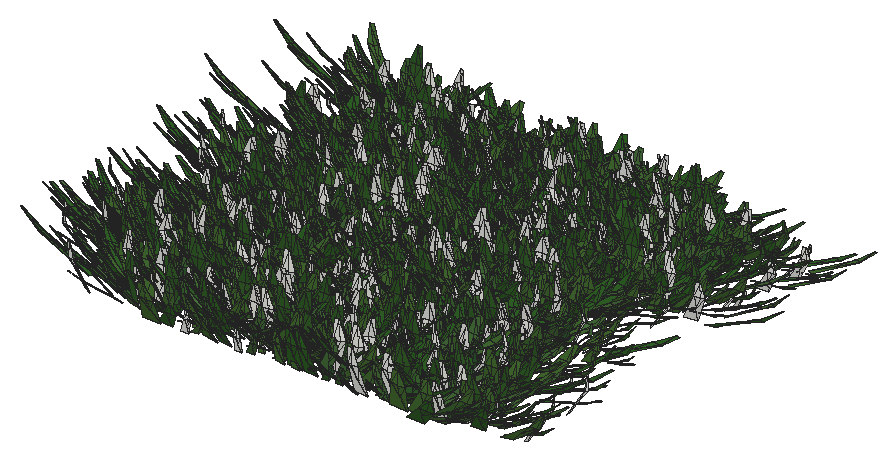
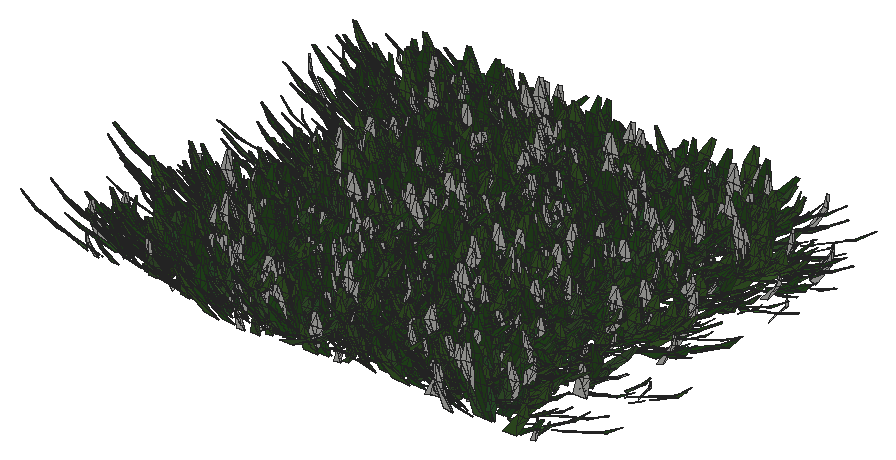
# SketchUp Ruby script. Lengths in inches.
U = 1.inch
M = Sketchup.active_model
def pt(a) = Geom::Point3d.new(a.map { |v| v * U })
def face(e, loops, mat)
  f = e.add_face(loops[0].map { |a| pt(a) })
  loops[1..].each { |l| e.add_face(l.map { |a| pt(a) }).erase! }
  f.material = f.back_material = mat if mat
  f
end
# faces: each face lists its corners as indices into pts; further lists are holes
def faces(e, pts, list, mat = nil) = list.each { |f| face(e, (f[0].is_a?(Array) ? f : [f]).map { |l| l.map { |i| pts[i] } }, mat) }
# xy, xz, yz: faces in a plane at the given z, y or x. An outline is a flat list of corners, or four numbers for a rectangle; further outlines are holes
def ring(l) = l.size == 4 ? [[l[0], l[1]], [l[2], l[1]], [l[2], l[3]], [l[0], l[3]]] : l.each_slice(2).to_a
def flat(e, list, mat, &to3) = list.each { |f| face(e, (f[0].is_a?(Array) ? f : [f]).map { |l| ring(l).map { |u, v| to3.(u, v) } }, mat) }
def xy(e, z, list, mat = nil) = flat(e, list, mat) { |x, y| [x, y, z] }
def xz(e, y, list, mat = nil) = flat(e, list, mat) { |x, z| [x, y, z] }
def yz(e, x, list, mat = nil) = flat(e, list, mat) { |y, z| [x, y, z] }
def lines(e, pts, list) = list.each { |a, b| e.add_line(pt(pts[a]), pt(pts[b])) }
# prism: a flat outline (further loops are holes) pulled along v
def prism(e, loops, v, mat = nil)
  f = face(e, loops, mat); d = Geom::Vector3d.new(v.map { |x| x * U })
  f.pushpull(f.normal.samedirection?(d) ? d.length : -d.length)
end
def box(e, o, s, mat = nil) = prism(e, [[o, [o[0] + s[0], o[1], o[2]], [o[0] + s[0], o[1] + s[1], o[2]], [o[0], o[1] + s[1], o[2]]]], [0, 0, s[2]], mat)
def at(x, y, z, deg = 0) = Geom::Transformation.translation(pt([x, y, z])) * Geom::Transformation.rotation(ORIGIN, Z_AXIS, deg.degrees)
def axes(o, x, y, z) = Geom::Transformation.new([*x, 0, *y, 0, *z, 0, *pt(o).to_a, 1])
def part(name) = M.definitions.add(name)
# library, detail: a bought-in or finely detailed component or shape, given as its bounding box
def library(name, o, s) = part(name).tap { |d| box(d.entities, o, s) }
def detail(e, o, s) = box(e.add_group.entities, o, s)
def put(e, d, t, mat = nil) = e.add_instance(d, t).tap { |i| i.material = mat if mat }
def group(e, t, mat = nil) = e.add_group.tap { |g| g.transformation = t; g.material = mat if mat }.entities
root = M.entities
M.materials.add("Material10").color = [48, 100, 38]
M.materials.add("Material3").color = [68, 110, 58]
M.materials.add("Material4").color = [48, 90, 38]
M.materials.add("Material5").color = [68, 110, 48]
M.materials.add("Material6").color = [48, 90, 48]
M.materials.add("Material7").color = [58, 110, 58]
M.materials.add("Material8").color = [58, 90, 38]
M.materials.add("Material9").color = [68, 100, 58]
c1 = part("grass00")
p = [[-0.6875,0.15,0],[-0.56,0.08,5.52],[-0.04,0.03,2.76],[0.48,-0.02,0],[0.35,-0.02,5.52],[-0.1,-0.14,5.52],
  [-0.12,0.65,8.37],[-0.42,0.65,8.37]]
faces(c1.entities,p,[[0,1,2,3],[3,2,4],[1,5,2],[5,4,2],[1,6,5],[4,5,6],[7,6,1]])
c2 = part("Group16\#1")
put(c2.entities,c1,axes([1.44,-0.61,-0.01],[0.05352,0.12609,0],[-0.10704,0.04543,0.07239],[0.06664,-0.02828,0.11628]),"Material6")
put(c2.entities,c1,axes([0.76,-0.15,-0.01],[0.04676,0.24062,0],[-0.23162,0.04501,0.06642],[0.0652,-0.01267,0.23595]),"Material3")
put(c2.entities,c1,axes([0.79,0.01,-0.01],[-0.00606,0.34651,0],[-0.34381,-0.00602,0.0432],[0.04319,0.00076,0.34386]))
put(c2.entities,c1,axes([1,0.23,-0.01],[-0.07192,0.31144,0],[-0.28722,-0.06632,0.1236],[0.12043,0.02781,0.29478]),"Material5")
put(c2.entities,c1,axes([1.66,0.77,-0.01],[-0.13828,0.29651,0],[-0.21551,-0.1005,0.22471],[0.20365,0.09498,0.23779]),"Material10")
put(c2.entities,c1,axes([0.6875,0.52,-0.01],[-0.18126,0.24051,0],[-0.22746,-0.17142,0.09788],[0.07817,0.05891,0.28481]),"Material5")
put(c2.entities,c1,axes([0.68,0.78,-0.01],[-0.215,0.18688,0],[-0.12385,-0.14248,0.21334],[0.13995,0.16101,0.18878]),"Material3")
put(c2.entities,c1,axes([0.56,1,-0.01],[-0.13756,0.07624,0],[-0.06159,-0.11112,0.0927],[0.04494,0.08108,0.12705]),"Material5")
put(c2.entities,c1,axes([0.2,0.64,-0.01],[-0.23729,0.07254,0],[-0.05711,-0.18681,0.153],[0.04473,0.14632,0.19535]),"Material10")
put(c2.entities,c1,axes([0.0625,0.72,-0.01],[-0.28874,0.02525,0],[-0.02179,-0.24916,0.14647],[0.01276,0.14591,0.25012]),"Material3")
put(c2.entities,c1,axes([-0.08,0.62,-0.01],[-0.34089,-0.04187,0],[0.03255,-0.26504,0.216],[-0.02633,0.21439,0.26703]),"Material10")
put(c2.entities,c1,axes([-0.34,0.98,-0.01],[-0.14314,-0.0493,0],[0.04397,-0.12769,0.06843],[-0.02228,0.0647,0.13505]),"Material10")
put(c2.entities,c1,axes([-0.87,1.45,-0.01],[-0.23488,-0.14114,0],[0.13761,-0.22901,0.06087],[-0.03135,0.05217,0.26717]))
put(c2.entities,c1,axes([-0.72,0.77,-0.01],[-0.14208,-0.13251,0],[0.07209,-0.0773,0.16301],[-0.11118,0.11922,0.1057]),"Material10")
put(c2.entities,c1,axes([-0.62,0.43,-0.01],[-0.14845,-0.21203,0],[0.18654,-0.13061,0.12304],[-0.10079,0.07057,0.22772]),"Material3")
put(c2.entities,c1,axes([-0.68,0.29,-0.01],[-0.13639,-0.32136,0],[0.31723,-0.13464,0.05579],[-0.05136,0.0218,0.34462]),"Material4")
put(c2.entities,c1,axes([-0.64,0.125,-0.01],[-0.0458,-0.23569,0],[0.22124,-0.043,0.08276],[-0.08124,0.01579,0.22538]),"Material7")
put(c2.entities,c1,axes([-1.6,-0.03,-0.01],[0.00576,-0.32897,0],[0.27526,0.00482,0.18018],[-0.18015,-0.00315,0.2753]),"Material5")
put(c2.entities,c1,axes([-1.36,-0.31,-0.01],[0.05718,-0.24765,0],[0.18172,0.04196,0.17267],[-0.16825,-0.03885,0.1865]),"Material10")
put(c2.entities,c1,axes([-1.54,-0.72,-0.01],[0.06537,-0.14017,0],[0.13555,0.06321,0.03939],[-0.0357,-0.01665,0.14956]))
put(c2.entities,c1,axes([-1.19,-0.9,-0.01],[0.09597,-0.12735,0],[0.11214,0.08451,0.07557],[-0.06035,-0.04548,0.14042]),"Material9")
put(c2.entities,c1,axes([-0.47,-0.54,-0.01],[0.11588,-0.10072,0],[0.0618,0.0711,0.12124],[-0.07953,-0.0915,0.0942]))
put(c2.entities,c1,axes([-0.47,-0.84,-0.01],[0.11927,-0.0661,0],[0.06603,0.11913,0.00646],[-0.00313,-0.00565,0.13621]),"Material5")
put(c2.entities,c1,axes([-0.38,-1.24,-0.01],[0.28037,-0.08571,0],[0.0618,0.20215,0.20315],[-0.05939,-0.19428,0.21139]),"Material9")
put(c2.entities,c1,axes([-0.06,-0.66,-0.01],[0.22719,-0.01987,0],[0.01247,0.14255,0.17758],[-0.01547,-0.17691,0.1431]),"Material8")
put(c2.entities,c1,axes([0.11,-0.89,-0.01],[0.14882,0.01828,0],[-0.01058,0.08611,0.12229],[0.01491,-0.12138,0.08676]),"Material6")
put(c2.entities,c1,axes([0.25,-0.72,-0.01],[0.20481,0.07053,0],[-0.06206,0.18022,0.10291],[0.03351,-0.0973,0.1906]),"Material6")
put(c2.entities,c1,axes([0.85,-1.42,-0.01],[0.16481,0.09904,0],[-0.09472,0.15762,0.05616],[0.02893,-0.04814,0.18389]),"Material5")
put(c2.entities,c1,axes([1.01,-1.09,-0.01],[0.21858,0.20385,0],[-0.17495,0.1876,0.15339],[0.10462,-0.11218,0.25652]),"Material10")
put(c2.entities,c1,axes([1.01,-0.71,-0.01],[0.08733,0.12473,0],[-0.06445,0.04512,0.13037],[0.1068,-0.07477,0.07867]),"Material6")
c3 = part("Group15\#1")
put(c3.entities,c2,at(0,0,0))
c4 = part("3darcstudiotree_grass00\#1")
put(c4.entities,c3,at(0,0,0))
put(root,c4,axes([955.85,939.92,0],[-0.75214,1.19237,0],[-4.74693,-0.18715,-0.03641],[-0.174,-0.00686,1.45326]))
put(root,c4,axes([955.95,963.41,0],[4.69551,-0.08423,0],[0.3605,1.25607,-0.01186],[0.0041,0.0143,1.52253]))
put(root,c4,axes([956.82,972.28,0],[2.38234,-0.95226,0],[3.20328,0.50086,-0.0272],[0.17769,0.02778,1.81972]))
put(root,c4,axes([956.31,940.49,0],[-1.46228,1.23307,0],[-3.47122,-0.25728,-0.00114],[-0.00907,-0.00067,1.86907]))
put(root,c4,axes([955.81,946.5,0],[1.47006,1.1325,0],[-4.40979,0.35776,-0.01715],[-0.07948,0.00645,1.41194]))
put(root,c4,axes([957,953.02,0],[-2.07415,0.83506,0],[-3.95028,-0.61324,-0.02009],[-0.09896,-0.01536,1.68525]))
put(root,c4,axes([957.88,954.94,0],[-1.18382,1.15457,0],[-4.70826,-0.30172,-0.05431],[-0.29177,-0.0187,1.6847]))
put(root,c4,axes([958.3,969.83,0],[-3.28461,0.98923,0],[-3.37325,-0.70003,-0.00469],[-0.02101,-0.00436,1.59556]))
put(root,c4,axes([957.74,956.29,0],[2.88148,0.64126,0],[-3.12484,0.87758,-0.03405],[-0.12784,0.0359,1.65877]))
put(root,c4,axes([958.03,942.36,0],[3.07935,0.60729,0],[-3.11371,0.98678,-0.06164],[-0.16424,0.05205,1.3518]))
put(root,c4,axes([958.4,937.74,0],[0.52678,1.06322,0],[-4.94177,0.15303,-0.03401],[-0.15238,0.00472,1.40523]))
put(root,c4,axes([960.7,959.67,0],[1.39418,-0.83958,0],[3.77377,0.39166,-0.03248],[0.18939,0.01966,1.61223]))
put(root,c4,axes([961.12,949.46,0],[-4.00371,0.05544,0],[-0.23957,-1.08136,-0.04105],[-0.01536,-0.06935,1.83253]))
put(root,c4,axes([960.22,961.01,0],[-0.74123,1.26839,0],[-3.97906,-0.14533,-0.03578],[-0.18887,-0.0069,1.34076]))
put(root,c4,axes([961.14,934.34,0],[-3.45273,0.48202,0],[-2.12645,-0.95198,-0.05669],[-0.18901,-0.08462,1.86391]))
put(root,c4,axes([961.79,942.36,0],[-2.58874,-0.9071,0],[3.15855,-0.56338,-0.04134],[0.26965,-0.0481,1.943]))
put(root,c4,axes([961,938.43,0],[-3.19228,0.66883,0],[-3.28024,-0.97852,-0.01682],[-0.06095,-0.01818,1.80026]))
put(root,c4,axes([961.375,964.91,0],[-3.68677,0.78294,0],[-2.37097,-0.69779,-0.00331],[-0.01382,-0.00407,1.47415]))
put(root,c4,axes([961.87,941.45,0],[2.79001,-0.91126,0],[3.28074,0.62779,-0.00025],[0.00114,0.00022,1.45509]))
put(root,c4,axes([961.69,951.44,0],[3.11012,-0.98955,0],[3.48139,0.68387,-0.04001],[0.20872,0.041,1.83572]))
put(root,c4,axes([960.94,947.1,0],[4.49844,0.3136,0],[-1.0523,0.94343,-0.03867],[-0.07449,0.06678,1.75619]))
put(root,c4,axes([961.3,966.6875,0],[0.32984,1.08986,0],[-4.10586,0.07766,-0.04286],[-0.23653,0.00447,1.42447]))
put(root,c4,axes([963.09,945.71,0],[-3.31262,-0.80999,0],[3.0672,-0.784,-0.0483],[0.19534,-0.04993,1.58573]))
put(root,c4,axes([962.21,968.11,0],[3.83987,-0.74679,0],[3.08152,0.9903,-0.05588],[0.18273,0.05872,1.67045]))
put(root,c4,axes([961.67,933.4,0],[-0.43739,1.1748,0],[-4.7805,-0.11124,-0.02425],[-0.1421,-0.00331,1.76617]))
put(root,c4,axes([963.72,970.83,0],[-1.00327,-1.08198,0],[4.89707,-0.2838,-0.01344],[0.05958,-0.00345,1.42931]))
put(root,c4,axes([962.97,957.125,0],[-4.17134,0.59694,0],[-1.91655,-0.83704,-0.03218],[-0.1099,-0.048,1.65786]))
put(root,c4,axes([963.5625,936.91,0],[1.82974,-1.11236,0],[4.14269,0.4259,-0.00107],[0.00497,0.00051,1.41133]))
put(root,c4,axes([962.8,969.7,0],[-2.1717,0.94775,0],[-3.61053,-0.51708,-0.00674],[-0.03293,-0.00472,1.46389]))
put(root,c4,axes([963.11,943.8,0],[-1.78952,0.96069,0],[-3.60864,-0.42012,-0.01596],[-0.10849,-0.01263,1.86544]))
put(root,c4,axes([963.37,948.01,0],[-2.06309,0.87153,0],[-4.13288,-0.61146,-0.04665],[-0.19777,-0.02926,1.47851]))
put(root,c4,axes([964.55,964.07,0],[-3.51429,-0.45659,0],[1.66461,-0.80077,-0.02241],[0.07721,-0.03714,1.68548]))
put(root,c4,axes([963.58,956.58,0],[2.73197,0.7121,0],[-2.97454,0.71324,-0.02632],[-0.14399,0.03453,1.95302]))
put(root,c4,axes([963.97,961.88,0],[4.48019,-0.41485,0],[1.31658,0.88866,-0.03178],[0.08406,0.05674,1.80429]))
put(root,c4,axes([963.76,939.38,0],[2.54094,0.64898,0],[-3.14239,0.76896,-0.01876],[-0.08636,0.02113,1.77063]))
put(root,c4,axes([964.56,952.54,0],[0.1997,1.06432,0],[-4.51312,0.05293,-0.04808],[-0.29009,0.0034,1.70557]))
put(root,c4,axes([963.97,955,0],[1.85724,1.07697,0],[-4.66485,0.50278,-0.01792],[-0.06948,0.00749,1.34035]))
put(root,c4,axes([966.91,963.85,0],[-1.0135,-1.00462,0],[4.08606,-0.25764,-0.02503],[0.13624,-0.00859,1.47852]))
put(root,c4,axes([966.41,943.59,0],[-4.005,0.7272,0],[-2.3018,-0.79231,-0.02785],[-0.12344,-0.04249,1.84622]))
put(root,c4,axes([966.39,951.57,0],[2.95335,-0.82152,0],[2.70823,0.6085,-0.01288],[0.06524,0.01466,1.54961]))
put(root,c4,axes([967.34,946.85,0],[-4.20956,-0.26717,0],[1.18231,-1.16431,-0.00944],[0.01496,-0.01473,1.93444]))
put(root,c4,axes([967.17,942.34,0],[-1.13661,-1.06386,0],[4.15271,-0.27729,-0.04991],[0.23787,-0.01588,1.32514]))
put(root,c4,axes([967.32,941.08,0],[2.16693,-1.10955,0],[3.94511,0.48154,-0.03421],[0.21213,0.02589,1.89316]))
put(root,c4,axes([966.46,953.29,0],[1.18,1.03822,0],[-4.57121,0.32472,-0.01918],[-0.11705,0.00831,1.88463]))
put(root,c4,axes([968.1,962.44,0],[-3.50507,0.61445,0],[-2.29769,-0.81919,-0.04222],[-0.17037,-0.06074,1.75818]))
put(root,c4,axes([969.18,959.26,0],[-3.58509,-0.60969,0],[2.592,-0.9526,-0.01911],[0.04957,-0.01822,1.32815]))
put(root,c4,axes([968.8125,939.43,0],[-0.06451,-0.92143,0],[4.54272,-0.01988,-0.04239],[0.21245,-0.00093,1.42343]))
put(root,c4,axes([968.87,965,0],[-4.03446,-0.01635,0],[0.06659,-1.02672,-0.00434],[0.00038,-0.00582,1.37632]))
put(root,c4,axes([967.4375,971.16,0],[3.92463,0.27646,0],[-1.34669,1.19487,-0.04858],[-0.06681,0.05928,1.57379]))
put(root,c4,axes([969.7,950.29,0],[-0.14207,-1.06089,0],[4.63971,-0.03883,-0.02714],[0.13515,-0.00113,1.44559]))
put(root,c4,axes([969.22,956.53,0],[-4.11295,0.48392,0],[-1.88318,-1.00036,-0.0027],[-0.00657,-0.00349,1.57765]))
put(root,c4,axes([969.27,969.92,0],[-3.01374,0.50325,0],[-2.28022,-0.85345,-0.04884],[-0.14675,-0.05493,1.38796]))
put(root,c4,axes([969.28,935.29,0],[2.85144,-0.93309,0],[3.29337,0.62902,-0.00592],[0.03247,0.0062,1.78738]))
put(root,c4,axes([970.22,936.01,0],[-2.85912,-0.7944,0],[3.18267,-0.71592,-0.02928],[0.11058,-0.02487,1.35967]))
put(root,c4,axes([970.48,967.84,0],[-4.01975,-0.67401,0],[2.06418,-0.76941,-0.03319],[0.1306,-0.04868,1.63594]))
put(root,c4,axes([969.0625,960.27,0],[-0.9226,1.08456,0],[-4.51637,-0.24012,-0.02719],[-0.16539,-0.00879,1.79436]))
put(root,c4,axes([969.36,954.06,0],[-0.15668,0.99341,0],[-4.74141,-0.04674,-0.01193],[-0.07952,-0.00078,1.97773]))
put(root,c4,axes([970.32,957.8,0],[-0.75974,1.09038,0],[-3.60462,-0.15698,-0.03897],[-0.29833,-0.01299,1.77692]))
put(root,c4,axes([970.2,945.88,0],[-0.10594,0.90385,0],[-3.73304,-0.02735,-0.04664],[-0.28296,-0.00207,1.41669]))
put(root,c4,axes([969.74,933.68,0],[1.08855,0.96574,0],[-4.18203,0.29461,-0.02067],[-0.12416,0.00875,1.69495]))
put(root,c4,axes([970.14,949.04,0],[3.05692,0.87665,0],[-2.75486,0.6004,-0.0286],[-0.17096,0.03726,1.81122]))
put(root,c4,axes([970.41,938.2,0],[-0.61059,1.1553,0],[-4.99702,-0.16506,-0.03274],[-0.14868,-0.00491,1.44297]))
put(root,c4,axes([970.23,966.68,0],[4.02977,0.69816,0],[-2.76519,0.99754,-0.01195],[-0.03084,0.01113,1.37528]))
put(root,c4,axes([972.49,959.14,0],[-4.6224,0.20326,0],[-0.67084,-0.9535,-0.03096],[-0.03075,-0.04371,1.38775]))
put(root,c4,axes([972.7,948.57,0],[-3.52473,0.27582,0],[-1.46531,-1.17033,-0.0251],[-0.03902,-0.03117,1.59541]))
put(root,c4,axes([973.27,969.67,0],[-3.34559,-0.54215,0],[2.26075,-0.87194,-0.04254],[0.15941,-0.06148,1.78955]))
put(root,c4,axes([972.73,957.2,0],[-3.01586,0.58588,0],[-3.13511,-1.00864,-0.03993],[-0.14863,-0.04782,1.9372]))
put(root,c4,axes([973.6875,961.8,0],[-4.50764,0.05804,0],[-0.237,-1.15033,-0.00589],[-0.00143,-0.00694,1.35922]))
put(root,c4,axes([972.76,939.04,0],[0.84914,1.0367,0],[-4.55233,0.23304,-0.02758],[-0.15102,0.00773,1.62317]))
put(root,c4,axes([974.6875,971.45,0],[0.34339,-1.17076,0],[3.77324,0.06917,-0.00239],[0.01439,0.00026,1.42634]))
put(root,c4,axes([973.05,949.6,0],[0.91899,1.10711,0],[-4.12174,0.21384,-0.00381],[-0.02297,0.00119,1.62105]))
put(root,c4,axes([974.92,965.39,0],[-4.49867,-0.03279,0],[0.10809,-0.92683,-0.0193],[0.00484,-0.04152,1.99558]))
put(root,c4,axes([974.98,945.13,0],[-5.14292,0.15234,0],[-0.50377,-1.06293,-0.03012],[-0.01728,-0.03646,1.30483]))
put(root,c4,axes([973.79,936.24,0],[-1.72517,0.88368,0],[-4.30295,-0.52503,-0.02753],[-0.1522,-0.01857,1.84121]))
put(root,c4,axes([974.21,938.3,0],[2.2537,-0.76087,0],[3.152,0.58351,-0.04843],[0.27401,0.05073,1.72564]))
put(root,c4,axes([974.97,967.69,0],[0.63611,-1.02473,0],[3.70027,0.14356,-0.00401],[0.03085,0.0012,1.82024]))
put(root,c4,axes([975.33,951.72,0],[1.35745,-0.83433,0],[3.74558,0.38088,-0.0011],[0.00732,0.00074,1.80895]))
put(root,c4,axes([975.39,943.83,0],[0.97823,-1.25703,0],[4.41558,0.21476,-0.02432],[0.13179,0.00641,1.55217]))
put(root,c4,axes([976.36,942.32,0],[0.22032,-0.95228,0],[4.21041,0.06088,-0.03098],[0.18429,0.00266,1.57088]))
put(root,c4,axes([976.88,954.93,0],[-3.97708,-0.65638,0],[2.24406,-0.84981,-0.0411],[0.12771,-0.04836,1.43569]))
put(root,c4,axes([976.74,941.48,0],[-0.40729,-1.01292,0],[4.15369,-0.10439,-0.02999],[0.21852,-0.00549,1.91089]))
put(root,c4,axes([976.44,952.76,0],[2.20159,-0.97329,0],[4.02139,0.56853,-0.04614],[0.20661,0.02921,1.48544]))
put(root,c4,axes([976.47,934.44,0],[3.52289,-0.91079,0],[3.16711,0.76564,-0.03201],[0.1577,0.03812,1.88682]))
put(root,c4,axes([975.98,964.03,0],[4.48262,0.00833,0],[-0.03164,1.06491,-0.04293],[-0.00162,0.05463,1.35522]))
put(root,c4,axes([976.5,955.54,0],[3.85076,-0.25069,0],[1.03247,0.9912,-0.03218],[0.04181,0.04014,1.32043]))
put(root,c4,axes([976.73,960.59,0],[3.89613,-0.16105,0],[0.82507,1.24749,-0.01648],[0.01292,0.01954,1.51991]))
put(root,c4,axes([976.88,967.07,0],[-0.04726,1.09729,0],[-5.17965,-0.01394,-0.05791],[-0.28781,-0.00077,1.60897]))
put(root,c4,axes([976.71,946.51,0],[5.05688,0.26305,0],[-1.05641,1.26926,-0.01168],[-0.01025,0.01231,1.39591]))
put(root,c4,axes([979.12,934.3,0],[2.70054,-0.71079,0],[3.38542,0.8039,-0.03691],[0.17495,0.04154,1.90749]))
put(root,c4,axes([980.18,950.27,0],[-3.16844,-0.68398,0],[2.56496,-0.74262,-0.01919],[0.10195,-0.02952,1.99409]))
put(root,c4,axes([978.41,971.55,0],[5.10235,-0.04118,0],[0.1288,0.99748,-0.01793],[0.00416,0.0322,1.79317]))
put(root,c4,axes([980.45,939.93,0],[-3.29965,-0.97084,0],[3.65156,-0.77567,-0.06095],[0.27313,-0.05802,1.76096]))
put(root,c4,axes([980.28,965.48,0],[0.00475,-1.00888,0],[4.13099,0.00122,-0.01884],[0.10616,0.00003,1.45492]))
put(root,c4,axes([980.28,942.82,0],[1.28562,-1.04456,0],[4.88305,0.37562,-0.02541],[0.11276,0.00867,1.48254]))
put(root,c4,axes([980.26,966.76,0],[-4.01095,0.48354,0],[-1.72258,-0.89306,-0.02015],[-0.06662,-0.03454,1.88684]))
put(root,c4,axes([981.04,946.94,0],[-4.2659,-0.35222,0],[1.33923,-1.01376,-0.04962],[0.10523,-0.07966,1.8049]))
put(root,c4,axes([980.36,941.33,0],[-3.11352,0.45479,0],[-2.39689,-1.02558,-0.05376],[-0.12618,-0.05399,1.38154]))
put(root,c4,axes([979.82,948.81,0],[-1.0061,1.18777,0],[-4.7987,-0.25405,-0.05285],[-0.29037,-0.01537,1.72177]))
put(root,c4,axes([981.42,972.35,0],[-1.74766,-0.79325,0],[4.51404,-0.62157,-0.06742],[0.28979,-0.0399,1.58058]))
put(root,c4,axes([980.65,954.47,0],[-3.06069,0.9303,0],[-3.81711,-0.78489,-0.01702],[-0.08141,-0.01674,1.91367]))
put(root,c4,axes([980.42,969.32,0],[4.53702,-0.3939,0],[1.61159,1.16016,-0.03586],[0.06911,0.04975,1.80381]))
put(root,c4,axes([980.62,936.55,0],[4.54274,-0.04809,0],[0.18784,1.10891,-0.02002],[0.00517,0.03055,1.69539]))
put(root,c4,axes([982.05,962.32,0],[-4.54396,0.24782,0],[-0.94268,-1.08027,-0.03649],[-0.05075,-0.05815,1.80375]))
put(root,c4,axes([980.59,958.83,0],[4.69542,0.51602,0],[-1.76105,1.00152,-0.02572],[-0.05567,0.03166,1.47108]))
put(root,c4,axes([982.65,945.04,0],[-4.19082,-0.16381,0],[0.77881,-1.24532,-0.04342],[0.03554,-0.05683,1.66984]))
put(root,c4,axes([981.48,952.84,0],[-2.14588,1.16725,0],[-4.21362,-0.48414,-0.02861],[-0.16909,-0.01943,1.88512]))
put(root,c4,axes([982.48,956.53,0],[-0.93459,-0.91429,0],[3.85666,-0.24639,-0.03508],[0.2611,-0.01668,1.91126]))
put(root,c4,axes([982.71,943.49,0],[-3.7798,-0.05998,0],[0.31505,-1.24085,-0.04372],[0.01169,-0.04605,1.31241]))
put(root,c4,axes([982.24,957.96,0],[-2.07802,0.79254,0],[-3.06125,-0.50166,-0.04],[-0.21333,-0.03496,1.45882]))
put(root,c4,axes([982.86,963.78,0],[-4.99575,0.35243,0],[-1.3345,-1.18231,-0.00145],[-0.00235,-0.00208,1.8291]))
put(root,c4,axes([981.64,968.56,0],[-0.1036,1.25235,0],[-5.07637,-0.02625,-0.04199],[-0.22282,-0.00115,1.68448]))
put(root,c4,axes([981.92,960.4,0],[4.03192,-0.06171,0],[0.31158,1.27245,-0.0507],[0.01617,0.06605,1.66388]))
put(root,c4,axes([982.05,951.5,0],[1.41099,1.21427,0],[-3.49838,0.25407,-0.00931],[-0.0535,0.00389,1.3628]))
put(root,c4,axes([982.89,938.39,0],[3.54443,-0.39661,0],[1.7308,0.96674,-0.04939],[0.13763,0.07687,1.80606]))
put(root,c4,axes([984.6875,957.77,0],[-3.31485,0.87666,0],[-3.1697,-0.74909,-0.01805],[-0.08242,-0.01948,1.71251]))
put(root,c4,axes([985.1875,953.24,0],[-3.48936,0.44199,0],[-1.76039,-0.8686,-0.00642],[-0.01577,-0.00778,1.3229]))
put(root,c4,axes([985.87,936.27,0],[-3.90886,-0.30229,0],[1.49188,-1.20572,-0.06046],[0.08426,-0.0681,1.48798]))
put(root,c4,axes([985.02,960.06,0],[-2.47789,0.67823,0],[-3.79555,-0.86668,-0.00484],[-0.01733,-0.00396,1.55938]))
put(root,c4,axes([985.37,934.74,0],[-3.37517,0.74484,0],[-3.41277,-0.96654,-0.01862],[-0.07294,-0.02066,1.90809]))
put(root,c4,axes([986.66,955.96,0],[-1.16922,-0.89242,0],[4.84591,-0.39681,-0.01545],[0.0714,-0.00585,1.54954]))
put(root,c4,axes([986.72,933.77,0],[-0.55416,-0.96725,0],[5.02165,-0.17981,-0.00214],[0.01069,-0.00038,1.59988]))
put(root,c4,axes([985.34,947.23,0],[-2.38604,0.77212,0],[-3.59178,-0.69372,-0.01374],[-0.06498,-0.01255,1.69563]))
put(root,c4,axes([984.97,939.625,0],[-1.2357,1.15486,0],[-4.4486,-0.2975,-0.00132],[-0.00824,-0.00055,1.858]))
put(root,c4,axes([984.54,951.63,0],[3.55659,0.85158,0],[-3.47186,0.90625,-0.01961],[-0.07165,0.0187,1.65716]))
put(root,c4,axes([986.57,937.8,0],[-4.00701,0.12184,0],[-0.61913,-1.27256,-0.00408],[-0.00269,-0.00553,1.74968]))
put(root,c4,axes([985.01,967.18,0],[0.70953,1.23995,0],[-4.73718,0.16942,-0.02596],[-0.11397,0.00408,1.32635]))
put(root,c4,axes([985.25,954.0625,0],[-1.18063,1.19799,0],[-4.72808,-0.29122,-0.00818],[-0.04761,-0.00293,1.82396]))
put(root,c4,axes([985.59,968.34,0],[2.66838,1.01095,0],[-3.09046,0.50982,-0.04277],[-0.24475,0.04038,1.58679]))
put(root,c4,axes([986.3,962.53,0],[4.51633,0.0703,0],[-0.2535,1.0179,-0.04181],[-0.01988,0.07984,1.95138]))
put(root,c4,axes([987.64,970.71,0],[-3.87975,0.70385,0],[-2.42692,-0.83611,-0.01293],[-0.05657,-0.01949,1.92389]))
put(root,c4,axes([986.27,949.54,0],[3.24301,0.83296,0],[-3.40593,0.82878,-0.004],[-0.01826,0.00444,1.89371]))
put(root,c4,axes([988.24,942.79,0],[-4.54194,0.17936,0],[-0.65445,-1.03581,-0.01239],[-0.01049,-0.01661,1.42361]))
put(root,c4,axes([986.87,940.99,0],[4.6124,0.10308,0],[-0.35679,0.99786,-0.01038],[-0.00716,0.02002,1.94021]))
put(root,c4,axes([986.88,959.07,0],[4.49423,0.49278,0],[-1.72551,0.98355,-0.04488],[-0.1327,0.07564,1.97665]))
put(root,c4,axes([987.01,944.2,0],[1.21551,1.05496,0],[-3.93123,0.28309,-0.02733],[-0.16885,0.01216,1.64375]))
put(root,c4,axes([988.15,969.41,0],[2.41626,-0.681,0],[3.66998,0.81384,-0.037],[0.13802,0.03061,1.52862]))
put(root,c4,axes([988.03,965.22,0],[2.63621,0.70043,0],[-2.68447,0.63147,-0.04643],[-0.25687,0.06042,1.7498]))
put(root,c4,axes([988.02,963.92,0],[2.03725,0.93622,0],[-3.24747,0.44167,-0.01685],[-0.12399,0.01686,1.93576]))
put(root,c4,axes([988.3,949.07,0],[4.58865,0.50519,0],[-1.59978,0.90817,-0.04159],[-0.09607,0.05454,1.42181]))
put(root,c4,axes([990.54,940.48,0],[-2.01574,-1.10957,0],[4.29176,-0.4873,-0.02239],[0.13134,-0.01491,1.89813]))
put(root,c4,axes([988.93,945.09,0],[1.09378,1.21386,0],[-4.24535,0.23909,-0.04632],[-0.26606,0.01498,1.6013]))
put(root,c4,axes([991.05,960.8,0],[-4.678,-0.23812,0],[0.97178,-1.1932,-0.03896],[0.04515,-0.05543,1.76791]))
put(root,c4,axes([990.7,959.5,0],[3.3432,-0.58816,0],[2.82496,1.00359,-0.04926],[0.17837,0.06337,1.93034]))
put(root,c4,axes([991.03,963.34,0],[-3.21056,0.58828,0],[-2.88924,-0.98552,-0.02359],[-0.07623,-0.026,1.66971]))
put(root,c4,axes([992.19,970.28,0],[-4.42597,-0.65302,0],[1.92536,-0.81559,-0.01139],[0.03728,-0.01579,1.52439]))
put(root,c4,axes([992.32,936.1875,0],[-0.4988,-1.1669,0],[3.78624,-0.10115,-0.01446],[0.09735,-0.0026,1.61179]))
put(root,c4,axes([991.71,935.25,0],[-3.42941,0.55901,0],[-2.40319,-0.92143,-0.02083],[-0.06645,-0.02548,1.60618]))
put(root,c4,axes([992.69,967.84,0],[-4.16493,-0.30995,0],[1.21489,-1.02032,-0.0137],[0.02048,-0.0172,1.39479]))
